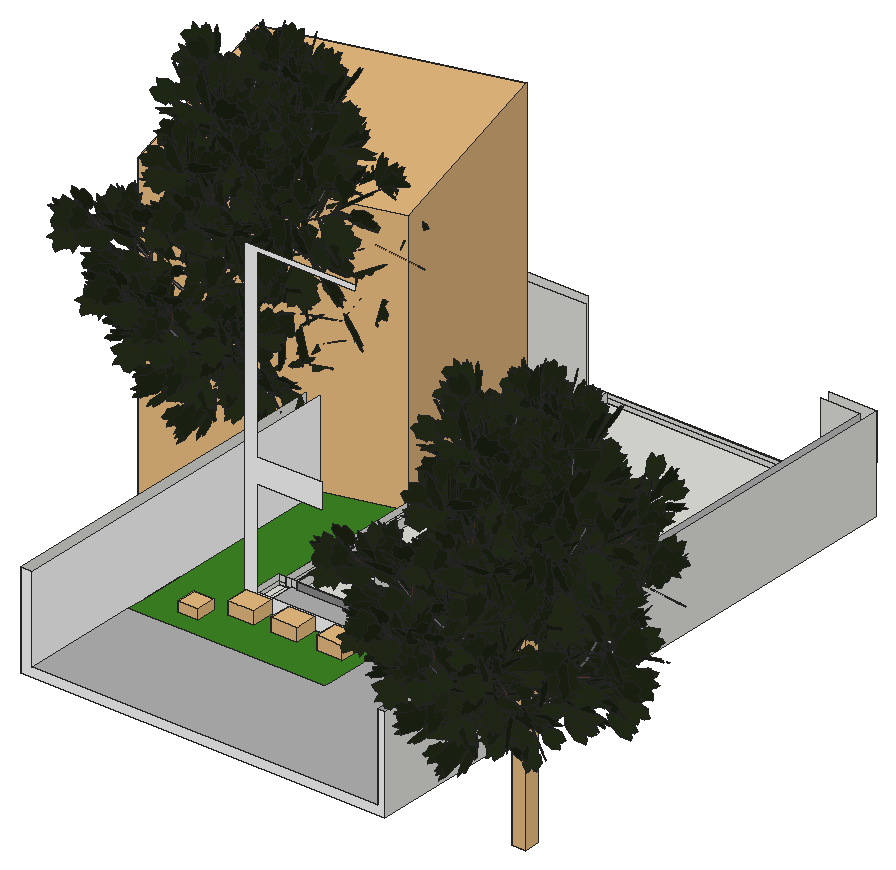
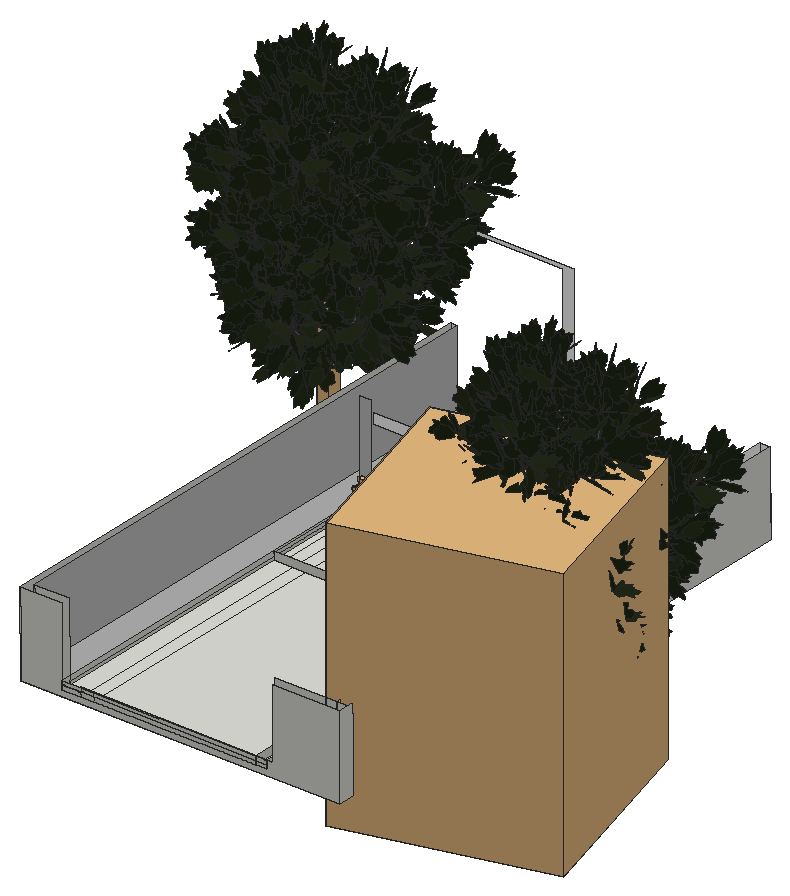
# SketchUp Ruby script. Lengths in inches.
U = 1.inch
M = Sketchup.active_model
def pt(a) = Geom::Point3d.new(a.map { |v| v * U })
def face(e, loops, mat)
  f = e.add_face(loops[0].map { |a| pt(a) })
  loops[1..].each { |l| e.add_face(l.map { |a| pt(a) }).erase! }
  f.material = f.back_material = mat if mat
  f
end
# faces: each face lists its corners as indices into pts; further lists are holes
def faces(e, pts, list, mat = nil) = list.each { |f| face(e, (f[0].is_a?(Array) ? f : [f]).map { |l| l.map { |i| pts[i] } }, mat) }
# xy, xz, yz: faces in a plane at the given z, y or x. An outline is a flat list of corners, or four numbers for a rectangle; further outlines are holes
def ring(l) = l.size == 4 ? [[l[0], l[1]], [l[2], l[1]], [l[2], l[3]], [l[0], l[3]]] : l.each_slice(2).to_a
def flat(e, list, mat, &to3) = list.each { |f| face(e, (f[0].is_a?(Array) ? f : [f]).map { |l| ring(l).map { |u, v| to3.(u, v) } }, mat) }
def xy(e, z, list, mat = nil) = flat(e, list, mat) { |x, y| [x, y, z] }
def xz(e, y, list, mat = nil) = flat(e, list, mat) { |x, z| [x, y, z] }
def yz(e, x, list, mat = nil) = flat(e, list, mat) { |y, z| [x, y, z] }
def lines(e, pts, list) = list.each { |a, b| e.add_line(pt(pts[a]), pt(pts[b])) }
# prism: a flat outline (further loops are holes) pulled along v
def prism(e, loops, v, mat = nil)
  f = face(e, loops, mat); d = Geom::Vector3d.new(v.map { |x| x * U })
  f.pushpull(f.normal.samedirection?(d) ? d.length : -d.length)
end
def box(e, o, s, mat = nil) = prism(e, [[o, [o[0] + s[0], o[1], o[2]], [o[0] + s[0], o[1] + s[1], o[2]], [o[0], o[1] + s[1], o[2]]]], [0, 0, s[2]], mat)
def at(x, y, z, deg = 0) = Geom::Transformation.translation(pt([x, y, z])) * Geom::Transformation.rotation(ORIGIN, Z_AXIS, deg.degrees)
def axes(o, x, y, z) = Geom::Transformation.new([*x, 0, *y, 0, *z, 0, *pt(o).to_a, 1])
def part(name) = M.definitions.add(name)
# library, detail: a bought-in or finely detailed component or shape, given as its bounding box
def library(name, o, s) = part(name).tap { |d| box(d.entities, o, s) }
def detail(e, o, s) = box(e.add_group.entities, o, s)
def put(e, d, t, mat = nil) = e.add_instance(d, t).tap { |i| i.material = mat if mat }
def group(e, t, mat = nil) = e.add_group.tap { |g| g.transformation = t; g.material = mat if mat }.entities
root = M.entities
M.materials.add("Green ash – green texture").color = [33, 41, 22]
M.materials.add("Moss 1").color = [97, 97, 43]
M.materials.add("[Color M00]").color = [255, 255, 255]
M.materials.add("[Color M02]").color = [198, 198, 198]
M.materials.add("[Color M03]").color = [170, 170, 170]
M.materials.add("[Color M04]").color = [60, 133, 34]
M.materials.add("[Color M04]1").color = [142, 142, 142]
M.materials.add("[Color_005]").color = [114, 114, 114]
M.materials.add("[Color_D09]").color = [86, 59, 49]
M.materials.add("[Groundcover_Wood_Mix]").color = [133, 121, 115]
M.materials.add("[Tile Grey]").color = [178, 178, 178]
M.materials.add("[Wood Veneer 01]").color = [120, 70, 37]
c1 = part("Component\#22")
xz(c1.entities,0,[[2.54,0,9.87,0.64,10.99,2.07,11.4,3.42,15.13,2.28,14.48,4.31,16.14,5.21,16.14,6.08,19.81,7.28,19.6,9.67,17.45,11.49,17.45,12.16,18.82,14.37,17.48,14.37,14.41,13.66,14.41,15.23,12.5625,17.49,9.84,15.21,8.9,13.85,7.74,13.625,7.35,12.68,6.87,13.02,6.35,12.27,5.92,10.47,4.2,7.42,2.84,6.89,0,2.38,0.07,1.59,2.8125,4.94,3.37,3.59,2.54,3.37,2.12,2.22]],"Green ash – green texture")
c2 = part("Component\#21")
xz(c2.entities,0,[[1.1,0,1.61,0,2.73,1.11,4.34,2.72,5.21,6.36,5.85,7.16,6.35,6.9375,6.85,8.05,8.03,8.05,8.625,9.25,10.11,11.7,9.56,13.83,9.56,15.84,7.83,15.84,6.03,14.37,5.31,16.54,4.4375,17.39,1.45,14.31,0,9.15,1.4,5.18,3.01,6.08,1.98,1.39]],"Green ash – green texture")
c3 = part("Component\#23")
put(c3.entities,c1,axes([0,7.77,0],[1,0,0],[0,0.89571,0.44464],[0,-0.44464,0.89571]))
put(c3.entities,c2,axes([2.15,6.37,5.26],[0.57629,-0.80824,0.12095],[0.79263,0.51673,-0.3236],[0.19905,0.28236,0.93843]))
c4 = part("Component\#24")
put(c4.entities,c3,axes([-4.97,-3.22,4.05],[0.69883,-0.69034,0.18725],[0.53248,0.3273,-0.7806],[0.47759,0.64522,0.59632]))
c5 = part("Component\#25")
put(c5.entities,c4,axes([0,5.2,2.2],[1,0,0],[0,0.90259,0.43051],[0,-0.43051,0.90259]))
c6 = part("leaf group 2")
put(c6.entities,c5,axes([-11.99,4.41,-4.35],[2.22014,-0.82385,1.14017],[1.36501,1.77637,-1.37441],[-0.33979,1.75315,1.92841]))
c7 = part("Component\#28")
put(c7.entities,c6,axes([-5.27,11.65,1.68],[-0.48323,0.10636,-0.43072],[-0.11515,-0.64511,-0.03012],[-0.42845,0.05342,0.49388]))
c8 = part("Component\#27")
xz(c8.entities,0,[[0.64,0,0,0.1875,4.21,2.81,8.59,4.11,12.8,4.11,19.57,2.81,12.8,3.73,8.59,3.73,4.21,2.3125]],"[Color_D09]")
c9 = part("Leaf cluster")
put(c9.entities,c7,axes([23.53,12.57,24.85],[0.06536,-0.90475,-0.42089],[0.61791,-0.2945,0.72901],[-0.78353,-0.30772,0.53981]))
put(c9.entities,c7,axes([22.7,12.25,24.83],[-0.47146,-0.89493,0.11311],[0.80135,-0.48549,-0.35888],[0.36776,-0.0521,0.90651]))
put(c9.entities,c7,axes([24.25,0.65,20.83],[0.8253,-0.50372,0.24924],[0.23848,0.71461,0.65749],[-0.51157,-0.48438,0.71194]))
put(c9.entities,c7,axes([23.54,-2.45,18.63],[0.04689,-0.92492,0.3511],[0.72122,-0.28285,-0.64421],[0.71641,0.2674,0.65188]))
put(c9.entities,c7,axes([22.39,16.15,27.04],[-0.5311,-0.82173,0.2419],[0.41574,0.01583,0.89559],[-0.77461,0.50499,0.40813]))
put(c9.entities,c8,axes([22.76,-5.09,13.48],[0,1.66539,0.44624],[-1.72414,0,0],[0,-0.44624,1.66539]))
c10 = part("Tree twig")
p = [[0,0,0.13],[0.41,0.77,0],[4.07,2.79,10.125],[3.73,2.15,10.23],[7.66,4.77,23.875],[7.4,4.27,23.96],
  [8.6875,5.26,35.99],[8.5,4.91,36.05],[8.32,4.9375,46.95],[8.21,4.74,46.98]]
faces(c10.entities,p,[[0,1,2,3],[3,2,4,5],[4,6,7,5],[6,8,9,7]],"[Color_005]")
c11 = part("Leafy twig")
put(c11.entities,c10,axes([3.13,0.17,-0.45],[3.38032,6.88592,0.52481],[-5.85488,3.97559,0.303],[0,-1.35912,3.54524]))
put(c11.entities,c7,axes([0.37,31.375,148.94],[0.47772,0.64064,-1.51139],[2.85768,-0.62659,0.20284],[-0.43926,-3.3797,-0.3241]))
c12 = part("Leafy branch")
put(c12.entities,c9,axes([28.11,72.66,46.26],[0.77413,-0.41274,-0.47998],[0.6311,0.56229,0.53435],[0.04934,-0.71657,0.69577]))
put(c12.entities,c9,axes([31.25,3.94,9.17],[0.73236,0.67893,0.05208],[-0.46223,0.55185,-0.69413],[-0.5,0.48428,0.71797]))
put(c12.entities,c9,axes([20.16,84.84,57.95],[0.96628,0.19619,0.16678],[-0.2575,0.73909,0.62245],[-0.00115,-0.6444,0.76469]))
put(c12.entities,c9,axes([30.13,29.18,11.93],[0.86603,0.2796,0.41452],[0,0.82904,-0.55919],[-0.5,0.48428,0.71797]))
put(c12.entities,c9,axes([47.67,28.63,-3.7],[0.1205,-0.71255,0.69119],[0.96646,0.24327,0.08231],[-0.2268,0.65809,0.71797]))
put(c12.entities,c9,axes([48.76,50.64,76.31],[-0.6716,0.46861,-0.57389],[0.01402,0.78248,0.62252],[0.74078,0.41004,-0.53209]))
put(c12.entities,c11,axes([42.34,0,10.34],[0.39368,0,0],[0,0.22544,-0.24092],[0,0.54032,0.50562]))
put(c12.entities,c9,axes([64.51,80.82,101.08],[-0.99604,0.06562,-0.06004],[-0.0106,0.58266,0.81265],[0.08831,0.81006,-0.57966]))
c13 = library("Tree trunk",[-6.35,9.4375,-76.57],[12.56,13.68,315.77])
c14 = part("Leafy branch \#2")
put(c14.entities,c9,axes([-3.64,36.17,23.18],[0.95801,0.10249,0.26779],[-0.28581,0.41631,0.86313],[-0.02302,-0.90343,0.42812]))
put(c14.entities,c9,axes([13.16,55.79,39.92],[0.70711,-0.61725,0.34497],[0,0.48786,0.87292],[-0.70711,-0.61725,0.34497]))
put(c14.entities,c11,axes([18.8125,5.17,0.46],[0.25503,0,0],[0,0.20007,-0.0752],[0,0.16866,0.44872]))
put(c14.entities,c9,axes([23.62,-10.17,21.5],[-0.56253,0.81775,0.12181],[0.38738,0.13053,0.91263],[0.73041,0.56057,-0.39021]))
put(c14.entities,c9,axes([45.18,27.18,68.96],[-0.96593,-0.22593,0.12627],[0.12295,0.02876,0.992],[-0.22775,0.97372,0]))
c15 = part("Leafy branch \#3")
put(c15.entities,c11,axes([21.47,3.93,0.22],[0.25503,0,0],[0,0.21068,-0.03601],[0,0.08077,0.47252]))
put(c15.entities,c9,axes([-4.05,13.6875,55.34],[0.70711,0.70373,-0.069],[0,0.09758,0.99523],[0.70711,-0.70373,0.069]))
put(c15.entities,c9,axes([6.52,33.54,18.07],[0.92587,-0.37604,0.03687],[0,0.09758,0.99523],[-0.37784,-0.92145,0.09035]))
c16 = part("Leafy branch \#1")
put(c16.entities,c9,axes([26.17,74.02,40.56],[0.25882,-0.64004,0.72344],[0,0.74896,0.66262],[-0.96593,-0.1715,0.19384]))
put(c16.entities,c9,axes([6.38,24.03,55.81],[-0.04786,0.8645,-0.50035],[0.15558,0.50126,0.85119],[0.98666,-0.03711,-0.15849]))
put(c16.entities,c11,axes([17.68,0,1.01],[0.32282,0,0],[0,0.21407,-0.16545],[0,0.37107,0.48011]))
put(c16.entities,c9,axes([-9.1875,31.15,28.07],[0.82314,0.37626,-0.42529],[0,0.74896,0.66262],[0.56784,-0.54543,0.61649]))
put(c16.entities,c9,axes([0.54,-12.07,9.94],[0.19622,0.90478,-0.37799],[-0.67396,0.40444,0.61823],[0.71224,0.13344,0.68914]))
put(c16.entities,c9,axes([7.34,9.15,39.57],[0.05153,0.73872,-0.67204],[0.38679,0.60565,0.6954],[0.92072,-0.29578,-0.25452]))
put(c16.entities,c9,axes([36.2,51.23,15.73],[-0.18626,-0.35374,0.91661],[-0.31641,0.90483,0.2849],[-0.93016,-0.23696,-0.28046]))
c17 = part("Tree")
put(c17.entities,c12,axes([-22.29,52.36,216.76],[0.38964,-1.07313,-0.10036],[1.06809,0.37236,0.19631],[-0.13881,-0.14712,1.22884]))
put(c17.entities,c12,axes([59.83,6.78,230.57],[-1.28826,-0.23008,-0.3647],[0.05148,-1.22938,0.51215],[-0.34663,0.55136,1.25774]))
put(c17.entities,c13,axes([-2.16,-18.04,104.22],[1.30157,0,0],[0,1.30157,0],[0,0,1.36111]))
put(c17.entities,c12,axes([-55.8,4.2,115.32],[1.30157,0,0],[0,1.29536,0.19359],[0,-0.26855,1.38538]))
put(c17.entities,c12,axes([5.36,-52.22,156.04],[-0.23532,1.19719,-0.71362],[-1.32974,0,0.39335],[0.40758,0.6912,1.23603]))
put(c17.entities,c14,axes([-20.09,22.57,317.7],[0,-1.33697,0],[1.33697,0,0],[0,0,1.4573]))
put(c17.entities,c12,axes([44.2,-31.84,172.82],[-1.11894,0.85085,0],[-0.85085,-1.11894,0],[0,0,1.53221]))
put(c17.entities,c12,axes([-10.2,63.7,119.93],[0.28716,-1.46366,0],[1.41378,0.27737,0.38604],[-0.41292,-0.08101,1.5704]))
put(c17.entities,c12,axes([-29.03,-40.72,232.79],[0.5211,0.98898,-0.38718],[-1.02974,0.58664,0.11255],[0.35577,0.28216,1.19957]))
put(c17.entities,c12,axes([44.92,21.7,135.38],[-1.05627,-0.44294,0],[0.44294,-1.05627,0],[0,0,1.24847]))
put(c17.entities,c14,axes([-32.94,-0.59,304.82],[1.2814,-0.22825,0],[0.22825,1.2814,0],[0,0,1.41871]))
put(c17.entities,c14,axes([0.6,-31.29,315.98],[0.13082,1.33422,0],[-1.33422,0.13082,0],[0,0,1.46127]))
put(c17.entities,c14,axes([21.3,1.66,315.16],[-1.25722,0.32198,-0.09905],[-0.32539,-1.26867,0.00612],[-0.08719,0.09194,1.40547]))
put(c17.entities,c15,axes([-19,30.84,372.72],[0.65078,-1.12719,0],[1.12719,0.65078,0],[0,0,1.41871]))
put(c17.entities,c15,axes([14.39,-16.125,357],[-0.73695,1.06095,0.15933],[-1.03698,-0.75397,0.2242],[0.29981,0,1.38667]))
put(c17.entities,c16,axes([-5.9,-20.03,270.39],[0,1.47598,0],[-1.4157,0,0.41751],[0.45509,0,1.54311]))
put(c17.entities,c16,axes([-18.4375,22.18,263.88],[0.84243,-1.42226,-0.32685],[1.40385,0.7063,0.64743],[-0.37678,-0.54841,1.68147]))
put(c17.entities,c16,axes([-29.32,4.9,283.41],[1.35363,0,0],[0,1.33841,0.20242],[0,-0.22063,1.45887]))
put(c17.entities,c16,axes([17.31,11.65,257.52],[-1.14969,-0.5642,-0.25322],[0.46017,-1.12719,0.50159],[-0.40066,0.32434,1.3027]))
put(c17.entities,c16,axes([16.3,15.3125,240.45],[-0.98541,-0.85203,0.68095],[1.00747,-1.01506,0.22317],[0.31818,0.5753,1.40228]))
put(c17.entities,c12,axes([-46.75,22.93,206.12],[1.08363,-0.37101,0],[0.37101,1.08363,0],[0,0,1.24847]))
put(c17.entities,c12,axes([41.1,-35.18,99.125],[-1.05556,0.85173,0.25344],[-0.84493,-1.04965,0.12953],[0.39153,-0.09409,1.38106]))
c18 = library("Palm tree",[-4.09,-4.52,0],[193.52,193.51,258.93])
c19 = part("Palm+Tree")
put(c19.entities,c18,at(25.51,-21.81,0,15))
c20 = library("Ornamental+Grasses",[-8.33,-8.78,0],[17.11,15.88,10.63])
c21 = part("HCD  9x9 Indo Pot (Square)")
xy(c21.entities,0,[[0,0,9,9]])
xy(c21.entities,0.75,[[0.75,0.75,8.25,8.25]])
xy(c21.entities,7.52,[[0.75,0.75,8.25,8.25]],"Moss 1")
xy(c21.entities,9,[[[0,0,9,9],[0.75,0.75,8.25,8.25]]])
xz(c21.entities,0,[[0,0,9,9]])
xz(c21.entities,0.75,[[0.75,0.75,8.25,7.52],[0.75,7.52,8.25,9]])
xz(c21.entities,8.25,[[0.75,0.75,8.25,7.52],[0.75,7.52,8.25,9]])
xz(c21.entities,9,[[0,0,9,9]])
yz(c21.entities,0,[[0,0,9,9]])
yz(c21.entities,0.75,[[0.75,0.75,8.25,7.52],[0.75,7.52,8.25,9]])
yz(c21.entities,8.25,[[0.75,0.75,8.25,7.52],[0.75,7.52,8.25,9]])
yz(c21.entities,9,[[0,0,9,9]])
c22 = part("Group\#284")
detail(c22.entities,[0,0,0],[2.15,3.79,14.3])
c23 = part("Potted plant")
put(c23.entities,c21,axes([7.375,7.93,0],[1.35,0,0],[0,1.35,0],[0,0,1.35]))
g1 = group(c23.entities,at(34.01,16.59,10.48),"[Groundcover_Wood_Mix]")
put(g1,c22,axes([-21.39,-3.67,0.04],[1.0831,1.67432,0],[1.44561,-0.94233,-0.44822],[0.5095,-0.33212,1.35364]))
put(g1,c22,axes([-19.2,-0.0625,0.04],[0.06577,-1.58752,0],[-1.23,-0.01362,-0.59477],[-0.71488,-0.00792,0.95418]))
put(g1,c22,axes([-20.16,-2.02,1.03],[1.23757,0.97175,0],[0.71987,-0.88743,-0.73204],[0.35645,-0.43942,0.56976]))
put(g1,c22,axes([-20.43,-4.53,0.04],[0.02652,1.58591,0],[1.23087,-0.05659,-0.59477],[0.71539,-0.03289,0.95418]))
put(g1,c22,axes([-19.73,-2.8125,1.03],[-1.55944,0.41251,0],[0.26154,1.08365,-0.73204],[0.12951,0.53658,0.56976]))
put(g1,c22,axes([-19.27,-4.42,0.04],[-1.00701,1.78126,0],[1.48381,0.79245,-0.44822],[0.52297,0.2793,1.35364]))
put(g1,c22,axes([-17.53,-1.6,0.04],[-1.30559,-0.8818,0],[-0.71402,1.01403,-0.59477],[-0.41499,0.58936,0.95418]))
put(g1,c22,axes([-21.8,-1.55,0.04],[2.03404,-0.13573,0],[-0.064,-1.68745,-0.44822],[-0.02256,-0.59474,1.35364]))
put(g1,c22,axes([-19.33,-2.61,1.03],[-1.22683,-0.98484,0],[-0.72899,0.88019,-0.73204],[-0.36097,0.43583,0.56976]))
put(g1,c22,axes([-19.3,-2.11,1.03],[0.27974,-1.57083,0],[-1.11549,-0.16277,-0.73204],[-0.55235,-0.0806,0.56976]))
put(g1,c22,axes([-21.97,-3.02,0.04],[1.31205,0.87256,0],[0.70701,-1.01874,-0.59477],[0.41092,-0.59209,0.95418]))
put(g1,c22,axes([-17.81,-3.69,0.04],[-1.51859,0.55236,0],[0.39363,1.14324,-0.59477],[0.22878,0.66446,0.95418]))
put(g1,c22,axes([-20.2,-2.52,1.03],[-0.299,1.5679,0],[1.11299,0.17632,-0.73204],[0.55111,0.08731,0.56976]))
put(g1,c22,axes([-21.28,-0.49,0.04],[1.33266,-0.92103,0],[-0.68389,-0.99325,-0.59477],[-0.39748,-0.57728,0.95418]))
put(g1,c22,axes([-19.17,-0.27,0.04],[-0.5456,-1.92548,0],[1.93945,-0.59168,-0.26656],[0.28985,-0.08843,1.78359]))
put(g1,c22,axes([-17.96,-1.15,0.04],[-1.27123,-1.53638,0],[-1.33347,1.09526,-0.44822],[-0.46998,0.38602,1.35364]))
put(g1,c22,axes([-19.65,-1.83,1.03],[1.43123,-0.75657,0],[-0.50987,-0.98658,-0.73204],[-0.25247,-0.48851,0.56976]))
put(g1,c22,axes([-16.8,-2.55,0.04],[-1.5632,-0.30402,0],[0.34989,-1.54112,-0.20989],[0.05229,-0.23032,1.4044]))
put(g1,c22,axes([-21.84,-2.79,0.04],[1.97107,0.44464,0],[-0.50241,1.94504,-0.26656],[-0.07509,0.29069,1.78359]))
put(g1,c22,axes([-20.37,0.56,0.04],[0.7463,-1.42646,0],[1.4028,0.68931,-0.20989],[0.20965,0.10302,1.4044]))
put(g1,c22,axes([-17.99,-3.6,0.04],[-1.66024,1.21511,0],[-1.16467,-1.59132,-0.26656],[-0.17406,-0.23783,1.78359]))
put(g1,c22,axes([-21.54,-4.58,0.04],[0.59386,1.45638,0],[-1.47231,0.6251,-0.20989],[-0.22004,0.09342,1.4044]))
put(g1,c22,axes([-19.92,-0.17,0.04],[0.74111,-1.89898,0],[-1.5902,-0.56846,-0.44822],[-0.56047,-0.20035,1.35364]))
c24 = library("Dome Light",[-12,-12,0],[24,24,12])
xy(root,49.27,[[331.5,348.42,612.66,449.29]])
xy(root,50.53,[[338.58,296.73,465.45,348.1],[465.45,296.73,480.01,348.1]])
xy(root,50.5625,[[331.5,348.42,346.7,449.29]])
xy(root,53.4375,[[480.01,345.98,505.26,348.85]],"[Wood Veneer 01]")
xy(root,56.49,[[480.01,345.98,505.26,348.85]],"[Wood Veneer 01]")
xy(root,57.25,[[480.01,345.98,505.26,349.54]],"[Wood Veneer 01]")
xy(root,58.21,[[505.26,346.79,506.42,352.35]],"[Color M03]")
xy(root,58.21,[[506.42,346.79,597.8,352.35]],"[Color M04]1")
xz(root,74.98,[[668.95,40.96,669.5,155.33,660.97,155.375,660.48,52.3125,245.97,54.28,246.46,157.34,232.71,157.41,232.17,43.03]],"[Color M00]")
xz(root,296.73,[[338.58,50.53,331.5,50.5625,331.5,50.83,338.58,50.82],[338.58,50.53,480.01,50.53,338.58,50.82],[480.01,50.53,480.01,51.03,338.58,51.03,338.58,50.82],[331.5,50.5625,323.37,50.6,323.375,50.85,331.5,50.83],[338.58,50.82,338.58,51.03,331.5,51.03,331.5,50.83],
  [331.5,50.83,331.5,51.03,323.375,51.03,323.375,50.85],[323.375,51.03,323.39,53.91,331.51,53.875,331.5,51.03],[331.5,51.03,331.51,53.875,338.59,53.84,338.58,51.03],[338.58,51.03,480.01,51.03,480.01,53.17,338.59,53.84]])
xz(root,296.73,[[480.01,53.17,480.01,148.12,480.06,148.88,480.21,149.63,480.45,150.35,480.79,151.04,481.22,151.68,481.72,152.25,482.3,152.76,482.93,153.18,483.62,153.52,484.34,153.77,485.09,153.92,485.86,153.97,597.79,153.97,597.79,168.47,486.52,168.47,483.77,168.29,481.07,167.75,478.46,166.86,475.99,165.64,473.69,164.11,471.625,162.3,469.81,160.23,468.28,157.93,467.06,155.46,466.17,152.85,465.63,150.15,465.45,147.4,465.45,94.23,465.25,91.1,464.64,88.01,463.625,85.04,462.24,82.22,460.49,79.61,458.42,77.25,456.06,75.18,453.45,73.43,450.63,72.04,447.66,71.03,444.57,70.42,441.44,70.22,338.58,70.22,338.58,186.3125,416.0625,186.3125,416.0625,215.9375,338.58,215.9375,338.58,435.25,456.36,435.25,456.36,441.25,323.43,441.25,323.43,61.75,323.39,53.91,331.51,53.875,338.59,53.84]],"[Color M00]")
xz(root,301.92,[[612.63,52.54,612.66,59.31,612.66,61.75,612.68,61.75,612.68,181.75,612.67,181.75,612.67,186.3125,597.79,186.3125,597.79,61.75,597.8,58.21,597.81,52.61,603.2,52.58]],"[Color M02]")
xz(root,345.98,[[480.01,53.4375,505.26,56.49],[480.01,57.25,505.26,60.3]],"[Wood Veneer 01]")
xz(root,346.79,[[586.68,49.35,586.7,52.66,597.81,52.61,597.8,58.21,505.26,58.21,505.26,61.75,480.01,61.75,480.01,61.04,346.76,61.68,346.7,50.5625,346.7,50.49,568.43,49.4375]],"[Color M04]1")
xz(root,348.1,[[586.68,49.35,568.43,49.4375,568.45,52.75,586.7,52.66],[568.43,49.4375,346.7,50.49,346.7,50.53,480.01,50.53,480.01,53.17,568.45,52.75],[346.7,50.49,338.58,50.53,346.7,50.53],[338.58,50.53,338.58,61.72,338.63,61.72,346.76,61.68,405.46,61.4,405.46,60.75,465.45,60.75,465.45,53.24,346.72,53.8,338.59,53.84],[338.58,50.53,338.59,53.84,346.72,53.8,346.7,50.5625,346.7,50.53],
  [346.7,50.53,346.7,50.5625,346.72,53.8,465.45,53.24,465.45,50.53],[465.45,50.53,465.45,53.24,480.01,53.17,480.01,50.53],[480.01,53.17,465.45,53.24,465.45,61.11,480.01,61.04]])
xz(root,348.42,[[612.62,49.23,603.18,49.27,612.62,49.27],[331.5,49.27,603.18,49.27,597.79,49.3,331.5,49.3],[603.18,49.27,603.2,52.58,597.81,52.61,597.79,49.3],[603.18,49.27,612.62,49.27,612.63,52.54,603.2,52.58],[612.62,49.27,612.66,49.27,612.66,59.31,612.63,52.54],
  [331.5,49.3,597.79,49.3,586.68,49.35,568.43,49.4375,346.7,50.49,338.58,50.53,331.5,50.5625],[597.79,49.3,597.81,52.61,586.7,52.66,586.68,49.35],[346.7,50.49,346.7,50.5625,338.58,50.5625,338.58,50.53],[338.58,50.53,338.58,50.5625,331.5,50.5625],[331.5,50.5625,323.37,50.6,323.39,53.91,331.5,53.875],
  [331.5,50.5625,331.51,53.875,331.5,53.875],[331.5,50.5625,338.58,50.5625,338.63,61.72,331.55,61.75,331.51,53.875],[338.58,50.5625,346.7,50.5625,346.7,61.68,338.63,61.72],[346.7,50.5625,346.76,61.68,346.7,61.68],[331.5,53.875,323.39,53.91,323.43,61.75,331.5,61.75],
  [331.5,53.875,331.51,53.875,331.55,61.75,331.5,61.75]])
xz(root,348.85,[[480.01,53.4375,505.26,56.49]],"[Wood Veneer 01]")
xz(root,349.54,[[480.01,57.25,505.26,60.3]],"[Wood Veneer 01]")
xz(root,352.35,[[505.26,58.21,597.8,58.21,597.79,61.75,505.26,61.75]],"[Color M04]1")
xz(root,449.29,[[331.5,49.27,331.5,50.5625,346.7,50.5625,346.7,60.48,597.79,60.48,612.66,60.41,612.66,49.27],[331.5,50.5625,346.7,60.48]])
xz(root,797.71,[[660.48,52.3125,660.97,155.375,613.12,155.6,612.68,61.75,612.67,60.41,612.63,52.54],[245.97,54.28,232.22,54.35,232.71,157.41,246.46,157.34]])
xz(root,811.1,[[668.95,40.96,232.17,43.03,232.71,157.41,323.43,156.98,323.43,61.75,331.55,61.75,331.5,50.5625,346.7,50.49,568.43,49.4375,586.68,49.35,612.62,49.23,612.65,55.54,612.65,55.625,612.67,60.41,612.68,61.75,613.12,155.6,669.5,155.33],[612.62,49.23,586.68,49.35,586.71,55.66,612.65,55.54],[586.68,49.35,568.43,49.4375,568.46,55.75,586.71,55.66],[568.43,49.4375,346.7,50.49,346.73,55.75,568.46,55.75],[346.7,50.49,331.5,50.5625,331.55,61.75,331.55,55.75,346.73,55.75],
  [612.65,55.54,586.71,55.66,586.71,55.75,586.74,55.75,612.65,55.625],[612.65,55.625,586.74,55.75,586.74,60.54,612.67,60.41],[586.71,55.66,568.46,55.75,586.71,55.75],[331.55,55.75,331.55,61.75,346.76,61.68,346.73,55.75],[586.71,55.75,586.74,60.54,568.49,60.625,480.01,60.625,480.01,61.04,346.76,61.68,331.55,61.75,586.74,61.75,586.74,55.75],
  [346.73,55.75,346.76,61.68,480.01,61.04,480.01,60.625,568.49,60.625,568.46,55.75],[568.46,55.75,568.49,60.625,586.74,60.54,586.71,55.75]])
yz(root,331.5,[[348.42,49.27,449.29,50.5625],[348.42,50.5625,449.29,61.75]])
yz(root,346.7,[[348.42,50.5625,449.29,61.75]])
yz(root,346.7,[[346.79,50.49,348.42,50.5625]],"[Color M03]")
yz(root,480.01,[[296.73,50.53,348.1,50.53,348.1,53.4375,345.98,53.4375,345.98,56.49,348.1,56.49,348.1,57.25,345.98,57.25,345.98,60.3,348.1,60.3,348.1,60.75,345.98,60.75,345.98,63.8,348.1,63.8,348.1,65.14,345.98,65.14,345.98,68.1875,348.1,68.1875,348.1,69.52,345.98,69.52,345.98,72.57,348.1,72.57,348.1,73.91,345.98,73.91,345.98,76.96,348.1,76.96,348.1,78.29,345.98,78.29,345.98,81.34,348.1,81.34,348.1,82.68,345.98,82.68,345.98,85.73,348.1,85.73,348.1,87.0625,345.98,87.0625,345.98,90.11,348.1,90.11,348.1,91.45,345.98,91.45,345.98,94.5,348.1,94.5,348.1,95.83,345.98,95.83,345.98,98.88,348.1,98.88,348.1,100.22,345.98,100.22,345.98,103.27,348.1,103.27,348.1,104.6,345.98,104.6,345.98,107.66,348.1,107.66,348.1,108.99,345.98,108.99,345.98,112.04,348.1,112.04,348.1,113.375,345.98,113.375,345.98,116.43,348.1,116.43,348.1,117.76,345.98,117.76,345.98,120.8125,348.1,120.8125,348.1,122.15,345.98,122.15,345.98,125.2,348.1,125.2,348.1,126.53,345.98,126.53,345.98,129.58,348.1,129.58,348.1,130.59,345.98,130.59,345.98,134.72,348.1,134.72,348.1,135.72,345.98,135.72,345.98,139.85,348.1,139.85,348.1,141.08,345.98,141.08,345.98,145.21,348.1,145.21,348.1,146.46,345.98,146.46,345.98,148.12,296.73,148.12],[345.98,53.4375,348.1,53.73],[345.98,53.73,348.1,53.8],[345.98,53.8,348.1,53.85],[345.98,53.85,348.1,54.4],
  [345.98,54.4,348.1,56.49],[345.98,57.25,348.1,57.54],[345.98,57.54,348.1,57.61],[345.98,57.61,348.1,57.67],[345.98,57.67,348.1,58.22],
  [345.98,58.22,348.1,60.3]])
yz(root,480.01,[[348.1,53.4375,348.85,53.73],[348.1,53.73,348.85,53.8],[348.1,53.8,348.85,53.85],[348.1,53.85,348.85,54.4],[348.1,54.4,348.85,56.49],
  [348.1,57.25,349.54,57.54],[348.1,57.54,349.54,57.61],[348.1,57.61,349.54,57.67],[348.1,57.67,349.54,58.22],[348.1,58.22,349.54,60.3]],"[Wood Veneer 01]")
yz(root,505.26,[[346.79,58.21,349.54,60.3],[349.54,58.21,352.35,60.3]],"[Color M03]")
yz(root,505.26,[[345.98,53.4375,348.42,56.49],[348.42,53.4375,348.85,56.49],[345.98,57.25,348.42,57.25,348.42,58.21,346.79,58.21,346.79,60.3,345.98,60.3],[348.42,57.25,349.54,58.21]],"[Wood Veneer 01]")
yz(root,612.66,[[348.42,49.27,449.29,49.27,449.29,60.625,301.92,60.625,301.92,59.31,348.42,59.31]])
p = [[232.17,811.1,43.03],[668.95,811.1,40.96],[668.95,74.98,40.96],[232.17,74.98,43.03],[669.5,811.1,155.33],[669.5,74.98,155.33],
  [232.71,811.1,157.41],[232.71,74.98,157.41],[232.71,797.71,157.41],[586.68,811.1,49.35],[586.68,348.42,49.35],[597.79,348.42,49.3],
  [603.18,348.42,49.27],[612.62,348.42,49.23],[612.62,797.71,49.23],[612.62,811.1,49.23],[612.63,797.71,52.54],[612.63,348.42,52.54],
  [612.62,348.42,49.27],[612.67,811.1,60.41],[612.67,797.71,60.41],[612.65,811.1,55.54],[612.65,811.1,55.625],[346.7,346.79,50.49],
  [346.7,348.1,50.49],[568.43,348.1,49.4375],[568.43,346.79,49.4375],[586.68,348.1,49.35],[586.68,346.79,49.35],[586.7,348.1,52.66],
  [586.7,346.79,52.66],[346.7,348.42,50.49],[568.43,348.42,49.4375],[586.7,348.42,52.66],[568.43,811.1,49.4375],[346.7,811.1,50.49],
  [346.7,449.29,50.49],[331.5,296.73,50.5625],[338.58,296.73,50.53],[338.58,348.1,50.53],[331.5,348.1,50.5625],[338.58,296.73,50.82],
  [338.58,296.73,51.03],[338.59,296.73,53.84],[338.59,348.1,53.84],[331.5,348.42,50.5625],[338.58,348.42,50.53],[331.5,449.29,50.5625],
  [346.7,348.42,50.5625],[346.73,811.1,55.75],[346.76,811.1,61.68],[346.76,449.29,61.68],[346.76,348.42,61.68],[331.5,811.1,50.5625],
  [331.5,798.27,50.5625],[323.37,348.1,50.6],[323.37,296.73,50.6],[323.375,296.73,50.85],[323.375,296.73,51.03],[323.39,296.73,53.91],
  [323.39,348.1,53.91],[346.7,348.1,50.5625],[346.7,346.79,50.5625],[346.76,346.79,61.68],[346.76,348.1,61.68],[323.37,348.42,50.6],
  [323.39,348.42,53.91],[331.51,348.42,53.875],[331.51,449.29,53.875],[331.51,798.27,53.875],[331.55,798.27,61.75],[331.55,811.1,61.75],
  [232.2,296.73,51.03],[232.2,240.6,51.03],[245.95,240.6,50.97],[245.95,296.73,50.97],[245.97,296.73,54.28],[245.97,240.6,54.28],
  [480.01,296.73,53.17],[481.16,296.73,53.16],[481.16,219.35,53.16],[245.97,219.35,54.28],[245.97,74.98,54.28],[660.48,74.98,52.3125],
  [660.48,797.71,52.3125],[612.63,301.92,52.54],[603.2,301.92,52.58],[597.81,301.92,52.61],[597.81,346.79,52.61],[568.45,348.1,52.75],
  [480.01,348.1,53.17],[465.45,348.1,53.24],[346.72,348.1,53.8],[660.97,797.71,155.375],[660.97,74.98,155.375],[603.2,348.42,52.58],
  [612.66,348.42,59.31],[612.66,301.92,59.31],[612.67,449.29,60.41],[612.67,348.42,60.41],[597.81,348.42,52.61],[597.8,301.92,58.21],
  [597.8,346.79,58.21],[331.51,296.73,53.875],[331.5,348.42,53.875],[232.22,797.71,54.35],[245.97,797.71,54.28],[323.43,296.73,61.75],
  [323.43,348.42,61.75],[331.55,348.42,61.75],[331.55,449.29,61.75],[332,798.27,156.9375],[246.46,74.98,157.34],[246.46,797.71,157.34],
  [597.79,301.92,61.75],[597.79,352.35,61.75],[597.8,352.35,58.21],[597.8,348.42,58.21],[232.2,296.73,50.53],[505.26,348.42,53.05],
  [505.26,348.42,53.4375],[505.26,348.42,56.49],[505.26,348.42,57.25],[597.95,348.42,58.21],[506.42,348.42,58.21],[506.42,348.42,53.04],
  [506.42,348.42,52.86]]
faces(root,p,[[0,1,2,3],[1,4,5,2],[6,0,3,7,8],[9,10,11,12,13,14,15],[13,14,16,17,18],[19,20,16,14,15,21,22],[31,32,25,24],[27,25,32,10],
  [27,10,33,29],[31,32,34,35,36],[34,32,10,9],[37,38,39,40],[39,38,41,42,43,44],[45,40,39,46],[39,40,45,46],[39,24,31,46],
  [47,45,46,31,36],[48,31,36,35,49,50,51,52],[53,54,47,36,35],[55,40,37,56],[55,56,57,58,59,60],[45,65,55,40],[65,55,60,66],[47,45,67,68],
  [47,68,69,54],[53,54,69,70,71],[72,73,74,75],[74,75,76,77],[16,20,98,99,96,17],[59,107,108,66,60],[70,69,68,67,109,110],[8,105,69,70,111]])
faces(root,p,[[23,24,25,26],[26,25,27,28],[28,27,29,30],[52,48,61,62,63,64],[17,95,86,85],[17,96,97,85],[95,100,88,87,86],[101,102,88,87],
  [100,33,29,30,88],[114,115,116,117,102,101]],"[Color M03]")
faces(root,p,[[44,43,78,79,80,81,82,83,84,16,17,85,86,87,88,30,29,89,90,91,92]],"[Tile Grey]")
faces(root,p,[[93,84,83,94]],"[Color M02]")
faces(root,p,[[103,59,60,66,104,67,68,69,105,106,76,77,81,80,79,78,43]],"[Color M04]")
faces(root,p,[[112,82,81,77,76,106,113]],"[Color M00]")
lines(root,p,[[118,72],[38,118],[119,120],[121,122],[117,123],[124,125],[125,126]])
put(root,c17,at(165.7,522.01,0))
put(root,c17,at(759.11,171.84,0))
put(root,c19,axes([34.01,497.25,0],[1.43,0,0],[0,1.43,0],[0,0,1.43]))
put(root,c20,axes([340.48,284.79,49.61],[1.81,0,0],[0,1.81,0],[0,0,1.81]))
put(root,c20,axes([392.04,284.79,49.61],[1.81,0,0],[0,1.81,0],[0,0,1.81]))
put(root,c20,axes([447.04,284.79,49.61],[1.81,0,0],[0,1.81,0],[0,0,1.81]))
put(root,c23,axes([573.42,298.71,52.76],[1.19,0,0],[0,1.19,0],[0,0,1.19]))
put(root,c24,at(298.65,255.34,54.03))
